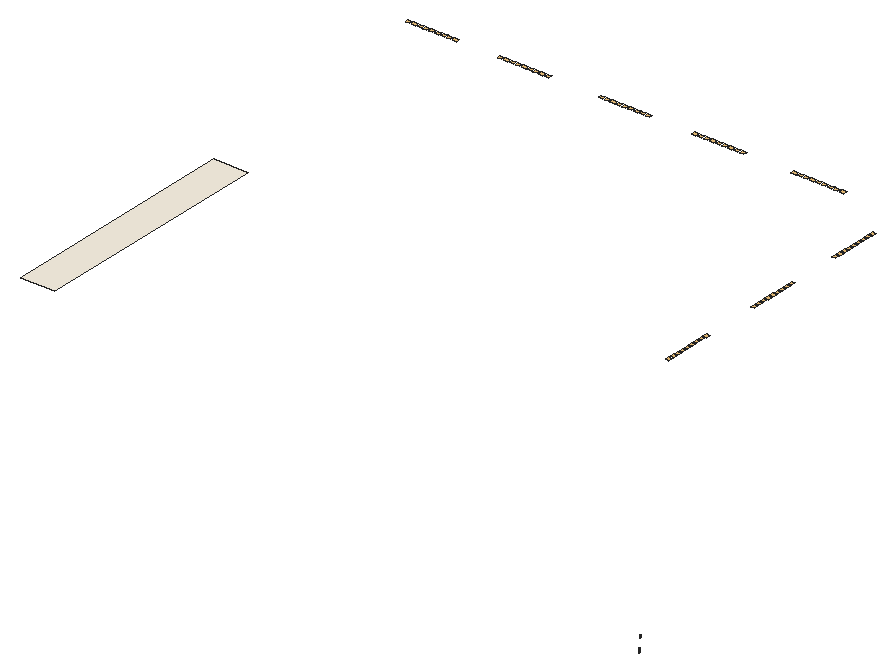
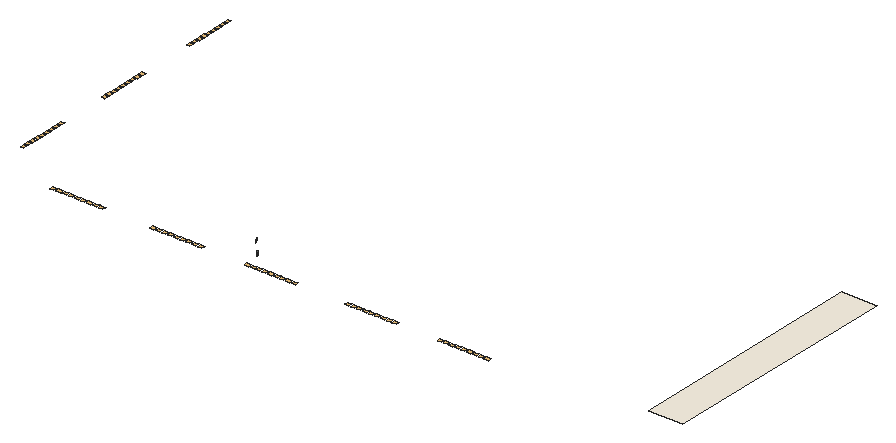
# SketchUp Ruby script. Lengths in inches.
U = 1.inch
M = Sketchup.active_model
def pt(a) = Geom::Point3d.new(a.map { |v| v * U })
def face(e, loops, mat)
  f = e.add_face(loops[0].map { |a| pt(a) })
  loops[1..].each { |l| e.add_face(l.map { |a| pt(a) }).erase! }
  f.material = f.back_material = mat if mat
  f
end
# faces: each face lists its corners as indices into pts; further lists are holes
def faces(e, pts, list, mat = nil) = list.each { |f| face(e, (f[0].is_a?(Array) ? f : [f]).map { |l| l.map { |i| pts[i] } }, mat) }
# xy, xz, yz: faces in a plane at the given z, y or x. An outline is a flat list of corners, or four numbers for a rectangle; further outlines are holes
def ring(l) = l.size == 4 ? [[l[0], l[1]], [l[2], l[1]], [l[2], l[3]], [l[0], l[3]]] : l.each_slice(2).to_a
def flat(e, list, mat, &to3) = list.each { |f| face(e, (f[0].is_a?(Array) ? f : [f]).map { |l| ring(l).map { |u, v| to3.(u, v) } }, mat) }
def xy(e, z, list, mat = nil) = flat(e, list, mat) { |x, y| [x, y, z] }
def xz(e, y, list, mat = nil) = flat(e, list, mat) { |x, z| [x, y, z] }
def yz(e, x, list, mat = nil) = flat(e, list, mat) { |y, z| [x, y, z] }
def lines(e, pts, list) = list.each { |a, b| e.add_line(pt(pts[a]), pt(pts[b])) }
# prism: a flat outline (further loops are holes) pulled along v
def prism(e, loops, v, mat = nil)
  f = face(e, loops, mat); d = Geom::Vector3d.new(v.map { |x| x * U })
  f.pushpull(f.normal.samedirection?(d) ? d.length : -d.length)
end
def box(e, o, s, mat = nil) = prism(e, [[o, [o[0] + s[0], o[1], o[2]], [o[0] + s[0], o[1] + s[1], o[2]], [o[0], o[1] + s[1], o[2]]]], [0, 0, s[2]], mat)
def at(x, y, z, deg = 0) = Geom::Transformation.translation(pt([x, y, z])) * Geom::Transformation.rotation(ORIGIN, Z_AXIS, deg.degrees)
def axes(o, x, y, z) = Geom::Transformation.new([*x, 0, *y, 0, *z, 0, *pt(o).to_a, 1])
def part(name) = M.definitions.add(name)
# library, detail: a bought-in or finely detailed component or shape, given as its bounding box
def library(name, o, s) = part(name).tap { |d| box(d.entities, o, s) }
def detail(e, o, s) = box(e.add_group.entities, o, s)
def put(e, d, t, mat = nil) = e.add_instance(d, t).tap { |i| i.material = mat if mat }
def group(e, t, mat = nil) = e.add_group.tap { |g| g.transformation = t; g.material = mat if mat }.entities
root = M.entities
M.materials.add("Material \#1").color = [140, 140, 140]
M.materials.add("[0030_OldLace]").color = [253, 245, 230]
M.materials.add("[Wood OSB]").color = [240, 195, 122]
xy(root,96,[[0,434.027,9,497.902]],"[0030_OldLace]")
xy(root,120,[[152.125,457.1,153,458.18],[152.125,458.647,153,459.726],[152.125,460.194,153,461.273],[152.125,461.741,153,462.82],[152.125,463.288,153,464.367],
  [152.125,464.834,153,465.914],[152.125,466.381,153,467.461],[152.125,467.928,153,469.008],[152.125,469.475,153,470.555],[152.125,485.35,153,486.43],
  [152.125,486.897,153,487.976],[152.125,488.444,153,489.523],[152.125,489.991,153,491.07],[152.125,491.538,153,492.617],[152.125,493.084,153,494.164],
  [152.125,494.631,153,495.711],[152.125,496.178,153,497.258],[152.125,497.725,153,498.805],[152.125,512.163,153,513.242],[152.125,513.709,153,514.789],
  [152.125,515.256,153,516.336],[152.125,516.803,153,517.883],[152.125,518.35,153,519.43],[152.125,519.897,153,520.976],[152.125,521.444,153,522.523],
  [152.125,522.991,153,524.07],[152.125,524.538,153,525.617],[21.405,534.59,22.484,535.465],[22.952,534.59,24.031,535.465],[24.499,534.59,25.578,535.465],
  [26.046,534.59,27.125,535.465],[27.592,534.59,28.672,535.465],[29.139,534.59,30.219,535.465],[30.686,534.59,31.766,535.465],[32.233,534.59,33.3125,535.465],
  [33.78,534.59,34.859,535.465],[45.717,534.59,46.797,535.465],[47.288,534.59,48.367,535.465],[48.858,534.59,49.9375,535.465],[50.428,534.59,51.508,535.465],
  [51.999,534.59,53.078,535.465],[53.569,534.59,54.649,535.465],[55.139,534.59,56.219,535.465],[56.71,534.59,57.789,535.465],[58.28,534.59,59.359,535.465],
  [72.405,534.59,73.484,535.465],[73.952,534.59,75.031,535.465],[75.499,534.59,76.578,535.465],[77.046,534.59,78.125,535.465],[78.592,534.59,79.672,535.465],
  [80.139,534.59,81.219,535.465],[81.686,534.59,82.766,535.465],[83.233,534.59,84.3125,535.465],[84.78,534.59,85.859,535.465],[97.155,534.59,98.234,535.465],
  [98.725,534.59,99.805,535.465],[100.296,534.59,101.375,535.465],[101.866,534.59,102.945,535.465],[103.436,534.59,104.516,535.465],[105.007,534.59,106.086,535.465],
  [106.577,534.59,107.656,535.465],[108.147,534.59,109.227,535.465],[109.717,534.59,110.797,535.465],[123.342,534.59,124.422,535.465],[124.944,534.59,126.024,535.465],
  [126.546,534.59,127.625,535.465],[128.147,534.59,129.227,535.465],[129.749,534.59,130.828,535.465],[131.35,534.59,132.43,535.465],[132.952,534.59,134.031,535.465],
  [134.553,534.59,135.633,535.465],[136.155,534.59,137.234,535.465]],"[Wood OSB]")
yz(root,155.634,[[444.023,57.44,444.023,57.481,443.974,57.489],[444.023,57.44,444.073,57.489,444.023,57.481],[444.023,57.44,444.079,57.449,444.131,57.475],[444.023,57.44,444.118,57.511,444.073,57.489],[444.023,57.44,444.131,57.475,444.214,57.568],
  [444.023,57.44,444.214,57.568,444.118,57.511],[444.131,57.475,444.176,57.516,444.214,57.568],[444.118,57.511,444.214,57.568,444.158,57.547],[444.023,57.513,444.023,57.524,443.973,57.523],[444.023,57.513,444.071,57.532,444.023,57.524],
  [444.023,57.513,444.073,57.523,444.071,57.532],[443.973,57.523,443.975,57.532,443.927,57.549],[443.973,57.523,444.023,57.524,443.975,57.532],[444.073,57.523,444.116,57.558,444.071,57.532],[444.073,57.523,444.12,57.549,444.116,57.558],
  [443.975,57.532,443.93,57.558,443.927,57.549],[444.158,57.547,444.214,57.568,444.192,57.594],[443.927,57.549,443.93,57.558,443.887,57.592],[444.12,57.549,444.154,57.599,444.116,57.558],[444.12,57.549,444.159,57.592,444.154,57.599],
  [443.93,57.558,443.892,57.599,443.887,57.592],[444.214,57.568,444.217,57.65,444.192,57.594],[444.214,57.568,444.234,57.713,444.217,57.65],[444.214,57.568,444.243,57.632,444.262,57.704],[444.214,57.568,444.262,57.704,444.266,57.827],
  [444.214,57.568,444.266,57.827,444.234,57.713],[443.887,57.592,443.892,57.599,443.856,57.648],[444.159,57.592,444.184,57.653,444.154,57.599],[444.159,57.592,444.19,57.648,444.184,57.653],[443.892,57.599,443.862,57.653,443.856,57.648],
  [443.856,57.648,443.862,57.653,443.837,57.712],[444.19,57.648,444.202,57.715,444.184,57.653],[444.19,57.648,444.209,57.712,444.202,57.715],[443.862,57.653,443.844,57.715,443.837,57.712],[444.262,57.704,444.268,57.782,444.266,57.827],
  [443.837,57.712,443.844,57.715,443.83,57.782],[444.209,57.712,444.209,57.782,444.202,57.715],[444.209,57.712,444.216,57.782,444.209,57.782],[444.234,57.713,444.266,57.827,444.239,57.782],[443.844,57.715,443.838,57.782,443.83,57.782],
  [443.83,57.782,443.838,57.782,443.837,57.852],[443.838,57.782,443.844,57.849,443.837,57.852],[444.209,57.782,444.216,57.782,444.202,57.849],[444.216,57.782,444.209,57.852,444.202,57.849],[444.239,57.782,444.266,57.827,444.234,57.851],
  [444.266,57.827,443.916,58.579,444.192,57.97],[444.266,57.827,444.165,58.066,443.916,58.579],[444.266,57.827,444.168,58.059,444.165,58.066],[444.266,57.827,444.172,58.053,444.168,58.059],[444.266,57.827,444.219,57.986,444.172,58.053],
  [444.266,57.827,444.192,57.97,444.217,57.914],[444.266,57.827,444.217,57.914,444.234,57.851],[444.266,57.827,444.25,57.912,444.219,57.986],[444.266,57.827,444.26,57.871,444.25,57.912],[443.844,57.849,443.856,57.916,443.837,57.852],
  [443.844,57.849,443.862,57.911,443.856,57.916],[444.202,57.849,444.209,57.852,444.184,57.911],[444.209,57.852,444.19,57.916,444.184,57.911],[443.862,57.911,443.887,57.972,443.856,57.916],[443.862,57.911,443.892,57.965,443.887,57.972],
  [444.184,57.911,444.19,57.916,444.154,57.965],[444.25,57.912,444.236,57.95,444.219,57.986],[444.19,57.916,444.159,57.972,444.154,57.965],[443.892,57.965,443.927,58.015,443.887,57.972],[443.892,57.965,443.93,58.006,443.927,58.015],
  [444.154,57.965,444.159,57.972,444.116,58.006],[444.192,57.97,443.916,58.579,444.158,58.017],[444.159,57.972,444.12,58.015,444.116,58.006],[444.219,57.986,444.177,58.047,444.172,58.053],[444.219,57.986,444.2,58.019,444.177,58.047],
  [443.93,58.006,443.973,58.041,443.927,58.015],[443.93,58.006,443.975,58.032,443.973,58.041],[444.116,58.006,444.12,58.015,444.071,58.032],[444.12,58.015,444.073,58.041,444.071,58.032],[444.158,58.017,443.916,58.579,444.118,58.053],
  [443.975,58.032,444.023,58.051,443.973,58.041],[443.975,58.032,444.023,58.04,444.023,58.051],[444.071,58.032,444.073,58.041,444.023,58.04],[444.023,58.04,444.073,58.041,444.023,58.051],[444.118,58.053,443.916,58.579,444.073,58.075],
  [444.165,58.066,444.163,58.073,443.916,58.579],[444.163,58.073,444.161,58.08,443.916,58.579],[444.073,58.075,443.916,58.579,444.023,58.083],[444.161,58.08,444.16,58.087,443.916,58.579],[444.16,58.087,444.13,58.579,443.916,58.579],
  [444.16,58.087,444.16,58.095,444.13,58.579],[444.16,58.095,444.157,58.504,444.13,58.579],[444.16,58.095,444.16,58.46,444.157,58.504],[444.157,58.504,444.146,58.544,444.13,58.579],[443.916,58.579,444.13,58.579,444.023,58.651],
  [444.13,58.579,444.083,58.631,444.023,58.651],[444.13,58.579,444.109,58.609,444.083,58.631],[444.083,58.631,444.055,58.646,444.023,58.651]],"Material \#1")
yz(root,155.637,[[444.643,60.789,444.654,60.79,444.633,60.951],[444.654,60.79,444.644,60.954,444.633,60.951],[444.633,60.951,444.644,60.954,444.604,61.097],[444.644,60.954,444.614,61.102,444.604,61.097],[444.204,61,444.22,61.045,444.209,61.051],
  [444.22,61.045,444.219,61.098,444.209,61.051],[444.22,61.045,444.229,61.095,444.219,61.098],[444.229,61.095,444.222,61.152,444.219,61.098],[444.229,61.095,444.233,61.152,444.222,61.152],[444.604,61.097,444.614,61.102,444.555,61.239],
  [444.614,61.102,444.564,61.246,444.555,61.239],[444.222,61.152,444.233,61.152,444.219,61.197],[444.233,61.152,444.229,61.199,444.219,61.197],[444.219,61.197,444.229,61.199,444.209,61.244],[444.229,61.199,444.22,61.249,444.209,61.244],
  [444.555,61.239,444.564,61.246,444.497,61.352],[444.564,61.246,444.505,61.361,444.497,61.352],[444.497,61.352,444.505,61.361,444.422,61.456],[444.505,61.361,444.429,61.467,444.422,61.456],[444.092,61.407,444.096,61.421,444.059,61.42],
  [444.059,61.42,444.096,61.421,444.061,61.434],[444.422,61.456,444.429,61.467,444.336,61.541],[444.429,61.467,444.341,61.554,444.336,61.541],[444.336,61.541,444.341,61.554,444.239,61.605],[444.341,61.554,444.243,61.619,444.239,61.605],
  [444.239,61.605,444.243,61.619,444.135,61.645],[444.243,61.619,444.137,61.66,444.135,61.645],[444.135,61.645,444.137,61.66,444.023,61.659]],"Material \#1")
